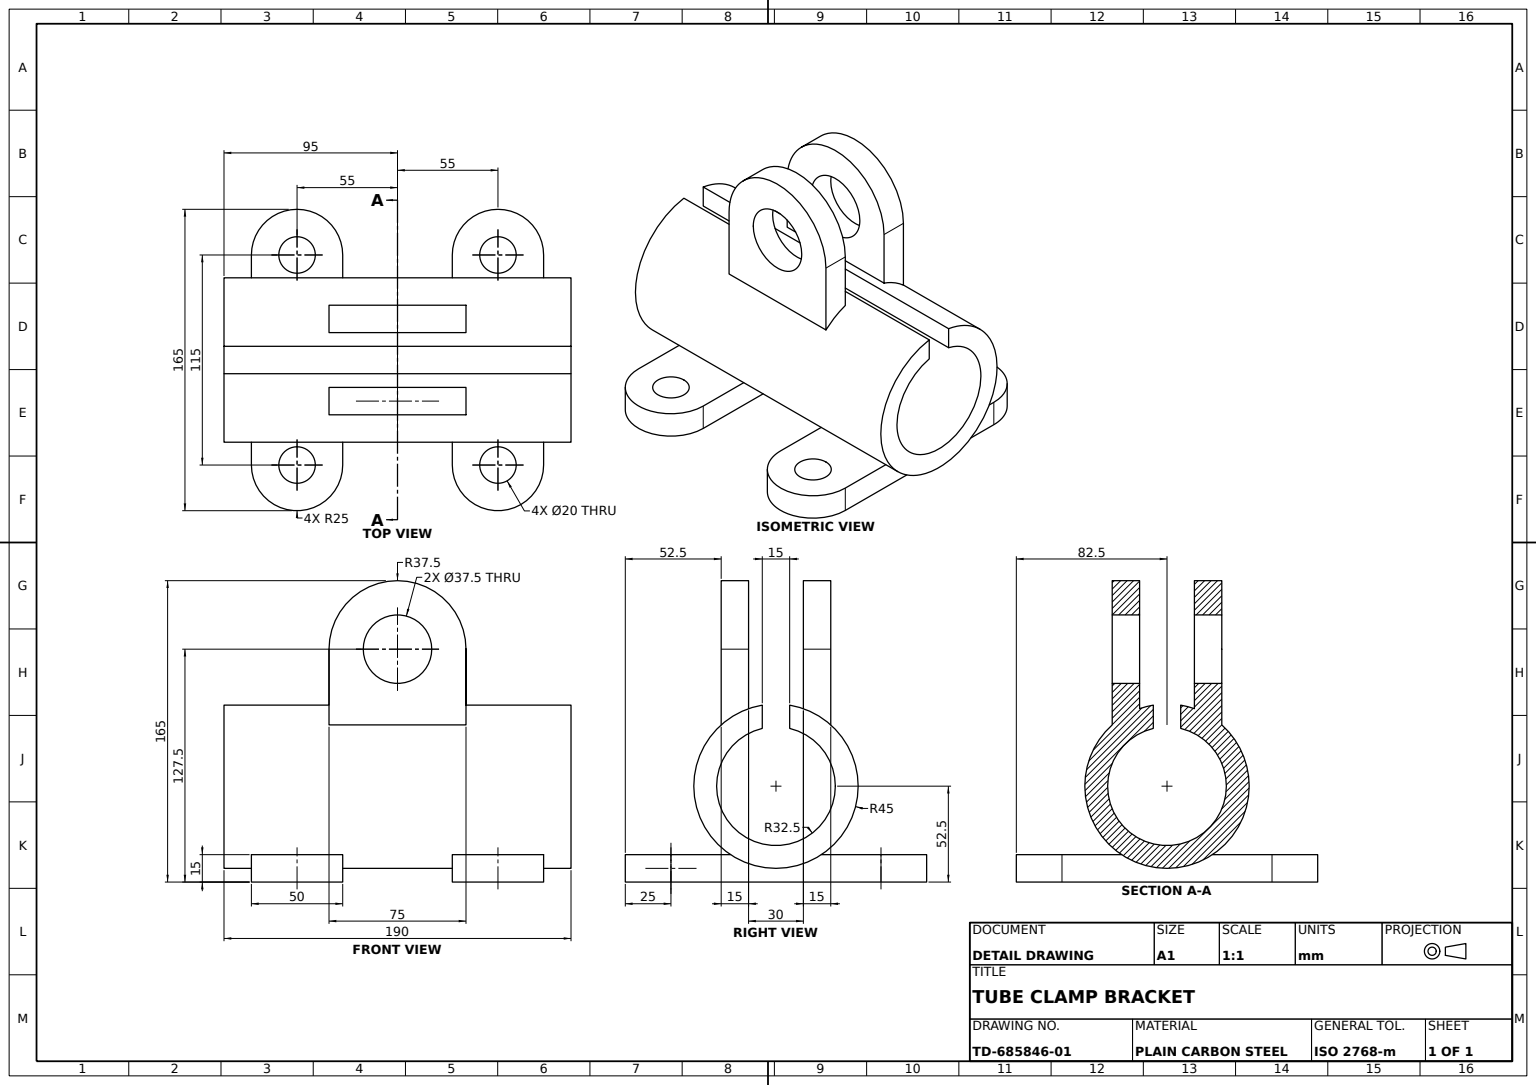
ISO-10303-21;
HEADER;
FILE_DESCRIPTION((''),'2;1');
FILE_NAME('','',(''),(''),'','','');
FILE_SCHEMA(('AUTOMOTIVE_DESIGN'));
ENDSEC;
DATA;
#1=APPLICATION_CONTEXT('');
#2=PRODUCT_CONTEXT('',#1,'mechanical');
#3=PRODUCT('','','',(#2));
#4=PRODUCT_DEFINITION_FORMATION('','',#3);
#5=PRODUCT_DEFINITION_CONTEXT('',#1,'design');
#6=PRODUCT_DEFINITION('','',#4,#5);
#7=PRODUCT_DEFINITION_SHAPE('','',#6);
#8=(LENGTH_UNIT()NAMED_UNIT(*)SI_UNIT(.MILLI.,.METRE.));
#9=(NAMED_UNIT(*)PLANE_ANGLE_UNIT()SI_UNIT($,.RADIAN.));
#10=(NAMED_UNIT(*)SI_UNIT($,.STERADIAN.)SOLID_ANGLE_UNIT());
#11=UNCERTAINTY_MEASURE_WITH_UNIT(LENGTH_MEASURE(1.E-05),#8,'distance_accuracy_value','');
#12=(GEOMETRIC_REPRESENTATION_CONTEXT(3)GLOBAL_UNCERTAINTY_ASSIGNED_CONTEXT((#11))GLOBAL_UNIT_ASSIGNED_CONTEXT((#8,#9,#10))REPRESENTATION_CONTEXT('',''));
#13=CARTESIAN_POINT('',(-55.,-37.5,67.5));
#14=VERTEX_POINT('',#13);
#15=CARTESIAN_POINT('',(-55.,-52.5,67.5));
#16=VERTEX_POINT('',#15);
#17=CARTESIAN_POINT('',(-55.,44.371598,67.5));
#18=DIRECTION('',(0.,-1.,0.));
#19=VECTOR('',#18,1000.);
#20=LINE('',#17,#19);
#21=EDGE_CURVE('',#14,#16,#20,.T.);
#22=ORIENTED_EDGE('',*,*,#21,.T.);
#23=CARTESIAN_POINT('',(-55.,-52.5,47.5));
#24=VERTEX_POINT('',#23);
#25=CARTESIAN_POINT('',(-55.,-52.5,57.5));
#26=DIRECTION('',(0.,0.,-1.));
#27=AXIS2_PLACEMENT_3D('',#25,#18,#26);
#28=CIRCLE('',#27,10.);
#29=EDGE_CURVE('',#16,#24,#28,.T.);
#30=ORIENTED_EDGE('',*,*,#29,.T.);
#31=CARTESIAN_POINT('',(-55.,-37.5,47.5));
#32=VERTEX_POINT('',#31);
#33=CARTESIAN_POINT('',(-55.,44.371598,47.5));
#34=LINE('',#33,#19);
#35=EDGE_CURVE('',#32,#24,#34,.T.);
#36=ORIENTED_EDGE('',*,*,#35,.F.);
#37=CARTESIAN_POINT('',(-55.,-37.5,57.5));
#38=DIRECTION('',(0.,1.,0.));
#39=AXIS2_PLACEMENT_3D('',#37,#38,#26);
#40=CIRCLE('',#39,10.);
#41=EDGE_CURVE('',#32,#14,#40,.T.);
#42=ORIENTED_EDGE('',*,*,#41,.T.);
#43=EDGE_LOOP('',(#22,#30,#36,#42));
#44=FACE_OUTER_BOUND('',#43,.T.);
#45=CARTESIAN_POINT('',(-55.,44.371598,57.5));
#46=AXIS2_PLACEMENT_3D('',#45,#18,#26);
#47=CYLINDRICAL_SURFACE('',#46,10.);
#48=ADVANCED_FACE('',(#44),#47,.F.);
#49=CARTESIAN_POINT('',(55.,-52.5,-82.5));
#50=VERTEX_POINT('',#49);
#51=CARTESIAN_POINT('',(80.,-52.5,-57.5));
#52=VERTEX_POINT('',#51);
#53=CARTESIAN_POINT('',(55.,-52.5,-57.5));
#54=AXIS2_PLACEMENT_3D('',#53,#18,#26);
#55=CIRCLE('',#54,25.);
#56=EDGE_CURVE('',#50,#52,#55,.T.);
#57=ORIENTED_EDGE('',*,*,#56,.T.);
#58=CARTESIAN_POINT('',(80.,-52.5,57.5));
#59=VERTEX_POINT('',#58);
#60=VECTOR('',#26,1000.);
#61=LINE('',#58,#60);
#62=EDGE_CURVE('',#59,#52,#61,.T.);
#63=ORIENTED_EDGE('',*,*,#62,.F.);
#64=CARTESIAN_POINT('',(30.,-52.5,57.5));
#65=VERTEX_POINT('',#64);
#66=CARTESIAN_POINT('',(55.,-52.5,57.5));
#67=DIRECTION('',(0.,0.,1.));
#68=AXIS2_PLACEMENT_3D('',#66,#38,#67);
#69=CIRCLE('',#68,25.);
#70=EDGE_CURVE('',#65,#59,#69,.T.);
#71=ORIENTED_EDGE('',*,*,#70,.F.);
#72=CARTESIAN_POINT('',(30.,-52.5,-57.5));
#73=VERTEX_POINT('',#72);
#74=LINE('',#64,#60);
#75=EDGE_CURVE('',#65,#73,#74,.T.);
#76=ORIENTED_EDGE('',*,*,#75,.T.);
#77=EDGE_CURVE('',#73,#50,#55,.T.);
#78=ORIENTED_EDGE('',*,*,#77,.T.);
#79=EDGE_LOOP('',(#57,#63,#71,#76,#78));
#80=FACE_OUTER_BOUND('',#79,.T.);
#81=CARTESIAN_POINT('',(55.,-52.5,-67.5));
#82=VERTEX_POINT('',#81);
#83=CARTESIAN_POINT('',(55.,-52.5,-47.5));
#84=VERTEX_POINT('',#83);
#85=CIRCLE('',#54,10.);
#86=EDGE_CURVE('',#82,#84,#85,.T.);
#87=ORIENTED_EDGE('',*,*,#86,.F.);
#88=EDGE_CURVE('',#84,#82,#85,.T.);
#89=ORIENTED_EDGE('',*,*,#88,.F.);
#90=EDGE_LOOP('',(#87,#89));
#91=FACE_BOUND('',#90,.T.);
#92=CARTESIAN_POINT('',(55.,-52.5,47.5));
#93=VERTEX_POINT('',#92);
#94=CARTESIAN_POINT('',(55.,-52.5,67.5));
#95=VERTEX_POINT('',#94);
#96=AXIS2_PLACEMENT_3D('',#66,#18,#26);
#97=CIRCLE('',#96,10.);
#98=EDGE_CURVE('',#93,#95,#97,.T.);
#99=ORIENTED_EDGE('',*,*,#98,.F.);
#100=EDGE_CURVE('',#95,#93,#97,.T.);
#101=ORIENTED_EDGE('',*,*,#100,.F.);
#102=EDGE_LOOP('',(#99,#101));
#103=FACE_BOUND('',#102,.T.);
#104=AXIS2_PLACEMENT_3D('',#58,#38,#67);
#105=PLANE('',#104);
#106=ADVANCED_FACE('',(#80,#91,#103),#105,.F.);
#107=CARTESIAN_POINT('',(-18.75,75.,-15.));
#108=VERTEX_POINT('',#107);
#109=CARTESIAN_POINT('',(18.75,75.,-15.));
#110=VERTEX_POINT('',#109);
#111=CARTESIAN_POINT('',(0.,75.,-15.));
#112=DIRECTION('',(1.,0.,0.));
#113=AXIS2_PLACEMENT_3D('',#111,#67,#112);
#114=CIRCLE('',#113,18.75);
#115=EDGE_CURVE('',#108,#110,#114,.T.);
#116=ORIENTED_EDGE('',*,*,#115,.F.);
#117=EDGE_CURVE('',#110,#108,#114,.T.);
#118=ORIENTED_EDGE('',*,*,#117,.F.);
#119=EDGE_LOOP('',(#116,#118));
#120=FACE_BOUND('',#119,.T.);
#121=CARTESIAN_POINT('',(37.5,75.,-15.));
#122=VERTEX_POINT('',#121);
#123=CARTESIAN_POINT('',(-37.5,75.,-15.));
#124=VERTEX_POINT('',#123);
#125=DIRECTION('',(-1.,0.,0.));
#126=AXIS2_PLACEMENT_3D('',#111,#67,#125);
#127=CIRCLE('',#126,37.5);
#128=EDGE_CURVE('',#122,#124,#127,.T.);
#129=ORIENTED_EDGE('',*,*,#128,.T.);
#130=CARTESIAN_POINT('',(-37.5,42.426407,-15.));
#131=VERTEX_POINT('',#130);
#132=LINE('',#123,#19);
#133=EDGE_CURVE('',#124,#131,#132,.T.);
#134=ORIENTED_EDGE('',*,*,#133,.T.);
#135=CARTESIAN_POINT('',(37.5,42.426407,-15.));
#136=VERTEX_POINT('',#135);
#137=CARTESIAN_POINT('',(95.,42.426407,-15.));
#138=VECTOR('',#125,1000.);
#139=LINE('',#137,#138);
#140=EDGE_CURVE('',#136,#131,#139,.T.);
#141=ORIENTED_EDGE('',*,*,#140,.F.);
#142=CARTESIAN_POINT('',(37.5,31.622777,-15.));
#143=VECTOR('',#38,1000.);
#144=LINE('',#142,#143);
#145=EDGE_CURVE('',#136,#122,#144,.T.);
#146=ORIENTED_EDGE('',*,*,#145,.T.);
#147=EDGE_LOOP('',(#129,#134,#141,#146));
#148=FACE_OUTER_BOUND('',#147,.T.);
#149=PLANE('',#126);
#150=ADVANCED_FACE('',(#120,#148),#149,.T.);
#151=CARTESIAN_POINT('',(80.,-37.5,-57.5));
#152=VERTEX_POINT('',#151);
#153=LINE('',#151,#143);
#154=EDGE_CURVE('',#52,#152,#153,.T.);
#155=ORIENTED_EDGE('',*,*,#154,.T.);
#156=CARTESIAN_POINT('',(80.,-37.5,-24.874686));
#157=VERTEX_POINT('',#156);
#158=CARTESIAN_POINT('',(80.,-37.5,57.5));
#159=LINE('',#158,#60);
#160=EDGE_CURVE('',#157,#152,#159,.T.);
#161=ORIENTED_EDGE('',*,*,#160,.F.);
#162=CARTESIAN_POINT('',(80.,-37.5,24.874686));
#163=VERTEX_POINT('',#162);
#164=CARTESIAN_POINT('',(80.,0.,0.));
#165=AXIS2_PLACEMENT_3D('',#164,#125,#67);
#166=CIRCLE('',#165,45.);
#167=EDGE_CURVE('',#157,#163,#166,.T.);
#168=ORIENTED_EDGE('',*,*,#167,.T.);
#169=VERTEX_POINT('',#158);
#170=EDGE_CURVE('',#169,#163,#159,.T.);
#171=ORIENTED_EDGE('',*,*,#170,.F.);
#172=LINE('',#158,#143);
#173=EDGE_CURVE('',#59,#169,#172,.T.);
#174=ORIENTED_EDGE('',*,*,#173,.F.);
#175=ORIENTED_EDGE('',*,*,#62,.T.);
#176=EDGE_LOOP('',(#155,#161,#168,#171,#174,#175));
#177=FACE_OUTER_BOUND('',#176,.T.);
#178=AXIS2_PLACEMENT_3D('',#158,#125,#67);
#179=PLANE('',#178);
#180=ADVANCED_FACE('',(#177),#179,.F.);
#181=CARTESIAN_POINT('',(-55.,-37.5,-67.5));
#182=VERTEX_POINT('',#181);
#183=CARTESIAN_POINT('',(-55.,-52.5,-67.5));
#184=VERTEX_POINT('',#183);
#185=CARTESIAN_POINT('',(-55.,44.371598,-67.5));
#186=LINE('',#185,#19);
#187=EDGE_CURVE('',#182,#184,#186,.T.);
#188=ORIENTED_EDGE('',*,*,#187,.F.);
#189=CARTESIAN_POINT('',(-55.,-37.5,-47.5));
#190=VERTEX_POINT('',#189);
#191=CARTESIAN_POINT('',(-55.,-37.5,-57.5));
#192=AXIS2_PLACEMENT_3D('',#191,#38,#26);
#193=CIRCLE('',#192,10.);
#194=EDGE_CURVE('',#182,#190,#193,.T.);
#195=ORIENTED_EDGE('',*,*,#194,.T.);
#196=CARTESIAN_POINT('',(-55.,-52.5,-47.5));
#197=VERTEX_POINT('',#196);
#198=CARTESIAN_POINT('',(-55.,44.371598,-47.5));
#199=LINE('',#198,#19);
#200=EDGE_CURVE('',#190,#197,#199,.T.);
#201=ORIENTED_EDGE('',*,*,#200,.T.);
#202=CARTESIAN_POINT('',(-55.,-52.5,-57.5));
#203=AXIS2_PLACEMENT_3D('',#202,#18,#26);
#204=CIRCLE('',#203,10.);
#205=EDGE_CURVE('',#197,#184,#204,.T.);
#206=ORIENTED_EDGE('',*,*,#205,.T.);
#207=EDGE_LOOP('',(#188,#195,#201,#206));
#208=FACE_OUTER_BOUND('',#207,.T.);
#209=CARTESIAN_POINT('',(-55.,44.371598,-57.5));
#210=AXIS2_PLACEMENT_3D('',#209,#18,#26);
#211=CYLINDRICAL_SURFACE('',#210,10.);
#212=ADVANCED_FACE('',(#208),#211,.F.);
#213=ORIENTED_EDGE('',*,*,#77,.F.);
#214=CARTESIAN_POINT('',(30.,-37.5,-57.5));
#215=VERTEX_POINT('',#214);
#216=LINE('',#214,#19);
#217=EDGE_CURVE('',#215,#73,#216,.T.);
#218=ORIENTED_EDGE('',*,*,#217,.F.);
#219=CARTESIAN_POINT('',(55.,-37.5,-82.5));
#220=VERTEX_POINT('',#219);
#221=CARTESIAN_POINT('',(55.,-37.5,-57.5));
#222=AXIS2_PLACEMENT_3D('',#221,#38,#26);
#223=CIRCLE('',#222,25.);
#224=EDGE_CURVE('',#220,#215,#223,.T.);
#225=ORIENTED_EDGE('',*,*,#224,.F.);
#226=CARTESIAN_POINT('',(55.,18.401699,-82.5));
#227=LINE('',#226,#19);
#228=EDGE_CURVE('',#220,#50,#227,.T.);
#229=ORIENTED_EDGE('',*,*,#228,.T.);
#230=EDGE_LOOP('',(#213,#218,#225,#229));
#231=FACE_OUTER_BOUND('',#230,.T.);
#232=CARTESIAN_POINT('',(55.,18.401699,-57.5));
#233=AXIS2_PLACEMENT_3D('',#232,#18,#26);
#234=CYLINDRICAL_SURFACE('',#233,25.);
#235=ADVANCED_FACE('',(#231),#234,.T.);
#236=ORIENTED_EDGE('',*,*,#98,.T.);
#237=CARTESIAN_POINT('',(55.,-37.5,67.5));
#238=VERTEX_POINT('',#237);
#239=CARTESIAN_POINT('',(55.,44.371598,67.5));
#240=LINE('',#239,#19);
#241=EDGE_CURVE('',#238,#95,#240,.T.);
#242=ORIENTED_EDGE('',*,*,#241,.F.);
#243=CARTESIAN_POINT('',(55.,-37.5,47.5));
#244=VERTEX_POINT('',#243);
#245=CARTESIAN_POINT('',(55.,-37.5,57.5));
#246=AXIS2_PLACEMENT_3D('',#245,#38,#26);
#247=CIRCLE('',#246,10.);
#248=EDGE_CURVE('',#238,#244,#247,.T.);
#249=ORIENTED_EDGE('',*,*,#248,.T.);
#250=CARTESIAN_POINT('',(55.,44.371598,47.5));
#251=LINE('',#250,#19);
#252=EDGE_CURVE('',#244,#93,#251,.T.);
#253=ORIENTED_EDGE('',*,*,#252,.T.);
#254=EDGE_LOOP('',(#236,#242,#249,#253));
#255=FACE_OUTER_BOUND('',#254,.T.);
#256=CARTESIAN_POINT('',(55.,44.371598,57.5));
#257=AXIS2_PLACEMENT_3D('',#256,#18,#26);
#258=CYLINDRICAL_SURFACE('',#257,10.);
#259=ADVANCED_FACE('',(#255),#258,.F.);
#260=ORIENTED_EDGE('',*,*,#115,.T.);
#261=CARTESIAN_POINT('',(18.75,75.,-30.));
#262=VERTEX_POINT('',#261);
#263=VECTOR('',#67,1000.);
#264=LINE('',#261,#263);
#265=EDGE_CURVE('',#262,#110,#264,.T.);
#266=ORIENTED_EDGE('',*,*,#265,.F.);
#267=CARTESIAN_POINT('',(-18.75,75.,-30.));
#268=VERTEX_POINT('',#267);
#269=CARTESIAN_POINT('',(0.,75.,-30.));
#270=AXIS2_PLACEMENT_3D('',#269,#67,#112);
#271=CIRCLE('',#270,18.75);
#272=EDGE_CURVE('',#268,#262,#271,.T.);
#273=ORIENTED_EDGE('',*,*,#272,.F.);
#274=LINE('',#267,#263);
#275=EDGE_CURVE('',#268,#108,#274,.T.);
#276=ORIENTED_EDGE('',*,*,#275,.T.);
#277=EDGE_LOOP('',(#260,#266,#273,#276));
#278=FACE_OUTER_BOUND('',#277,.T.);
#279=CYLINDRICAL_SURFACE('',#270,18.75);
#280=ADVANCED_FACE('',(#278),#279,.F.);
#281=CARTESIAN_POINT('',(30.,-37.5,24.874686));
#282=VERTEX_POINT('',#281);
#283=CARTESIAN_POINT('',(95.,-37.5,24.874686));
#284=LINE('',#283,#138);
#285=EDGE_CURVE('',#163,#282,#284,.T.);
#286=ORIENTED_EDGE('',*,*,#285,.T.);
#287=CARTESIAN_POINT('',(30.,-37.5,57.5));
#288=VERTEX_POINT('',#287);
#289=LINE('',#287,#60);
#290=EDGE_CURVE('',#288,#282,#289,.T.);
#291=ORIENTED_EDGE('',*,*,#290,.F.);
#292=AXIS2_PLACEMENT_3D('',#245,#18,#26);
#293=CIRCLE('',#292,25.);
#294=EDGE_CURVE('',#169,#288,#293,.T.);
#295=ORIENTED_EDGE('',*,*,#294,.F.);
#296=ORIENTED_EDGE('',*,*,#170,.T.);
#297=EDGE_LOOP('',(#286,#291,#295,#296));
#298=FACE_OUTER_BOUND('',#297,.T.);
#299=EDGE_CURVE('',#244,#238,#247,.T.);
#300=ORIENTED_EDGE('',*,*,#299,.F.);
#301=ORIENTED_EDGE('',*,*,#248,.F.);
#302=EDGE_LOOP('',(#300,#301));
#303=FACE_BOUND('',#302,.T.);
#304=AXIS2_PLACEMENT_3D('',#158,#18,#26);
#305=PLANE('',#304);
#306=ADVANCED_FACE('',(#298,#303),#305,.F.);
#307=CARTESIAN_POINT('',(95.,44.370598,-7.5));
#308=VERTEX_POINT('',#307);
#309=CARTESIAN_POINT('',(-95.,44.370598,-7.5));
#310=VERTEX_POINT('',#309);
#311=LINE('',#307,#138);
#312=EDGE_CURVE('',#308,#310,#311,.T.);
#313=ORIENTED_EDGE('',*,*,#312,.F.);
#314=CARTESIAN_POINT('',(95.,0.,-45.));
#315=VERTEX_POINT('',#314);
#316=CARTESIAN_POINT('',(95.,0.,0.));
#317=AXIS2_PLACEMENT_3D('',#316,#112,#67);
#318=CIRCLE('',#317,45.);
#319=EDGE_CURVE('',#315,#308,#318,.T.);
#320=ORIENTED_EDGE('',*,*,#319,.F.);
#321=CARTESIAN_POINT('',(-95.,0.,-45.));
#322=VERTEX_POINT('',#321);
#323=LINE('',#314,#138);
#324=EDGE_CURVE('',#315,#322,#323,.T.);
#325=ORIENTED_EDGE('',*,*,#324,.T.);
#326=CARTESIAN_POINT('',(-95.,0.,0.));
#327=AXIS2_PLACEMENT_3D('',#326,#112,#67);
#328=CIRCLE('',#327,45.);
#329=EDGE_CURVE('',#322,#310,#328,.T.);
#330=ORIENTED_EDGE('',*,*,#329,.T.);
#331=EDGE_LOOP('',(#313,#320,#325,#330));
#332=FACE_OUTER_BOUND('',#331,.T.);
#333=CARTESIAN_POINT('',(37.5,33.54102,-30.));
#334=VERTEX_POINT('',#333);
#335=CARTESIAN_POINT('',(37.5,0.,0.));
#336=AXIS2_PLACEMENT_3D('',#335,#112,#26);
#337=CIRCLE('',#336,45.);
#338=EDGE_CURVE('',#334,#136,#337,.T.);
#339=ORIENTED_EDGE('',*,*,#338,.T.);
#340=ORIENTED_EDGE('',*,*,#140,.T.);
#341=CARTESIAN_POINT('',(-37.5,33.54102,-30.));
#342=VERTEX_POINT('',#341);
#343=CARTESIAN_POINT('',(-37.5,0.,0.));
#344=AXIS2_PLACEMENT_3D('',#343,#125,#67);
#345=CIRCLE('',#344,45.);
#346=EDGE_CURVE('',#131,#342,#345,.T.);
#347=ORIENTED_EDGE('',*,*,#346,.T.);
#348=CARTESIAN_POINT('',(95.,33.54102,-30.));
#349=LINE('',#348,#138);
#350=EDGE_CURVE('',#334,#342,#349,.T.);
#351=ORIENTED_EDGE('',*,*,#350,.F.);
#352=EDGE_LOOP('',(#339,#340,#347,#351));
#353=FACE_BOUND('',#352,.T.);
#354=AXIS2_PLACEMENT_3D('',#316,#125,#67);
#355=CYLINDRICAL_SURFACE('',#354,45.);
#356=ADVANCED_FACE('',(#332,#353),#355,.T.);
#357=ORIENTED_EDGE('',*,*,#41,.F.);
#358=EDGE_CURVE('',#14,#32,#40,.T.);
#359=ORIENTED_EDGE('',*,*,#358,.F.);
#360=EDGE_LOOP('',(#357,#359));
#361=FACE_BOUND('',#360,.T.);
#362=CARTESIAN_POINT('',(-80.,-37.5,57.5));
#363=VERTEX_POINT('',#362);
#364=CARTESIAN_POINT('',(-80.,-37.5,24.874686));
#365=VERTEX_POINT('',#364);
#366=LINE('',#362,#60);
#367=EDGE_CURVE('',#363,#365,#366,.T.);
#368=ORIENTED_EDGE('',*,*,#367,.F.);
#369=CARTESIAN_POINT('',(-30.,-37.5,57.5));
#370=VERTEX_POINT('',#369);
#371=CIRCLE('',#39,25.);
#372=EDGE_CURVE('',#363,#370,#371,.T.);
#373=ORIENTED_EDGE('',*,*,#372,.T.);
#374=CARTESIAN_POINT('',(-30.,-37.5,24.874686));
#375=VERTEX_POINT('',#374);
#376=LINE('',#369,#60);
#377=EDGE_CURVE('',#370,#375,#376,.T.);
#378=ORIENTED_EDGE('',*,*,#377,.T.);
#379=EDGE_CURVE('',#375,#365,#284,.T.);
#380=ORIENTED_EDGE('',*,*,#379,.T.);
#381=EDGE_LOOP('',(#368,#373,#378,#380));
#382=FACE_OUTER_BOUND('',#381,.T.);
#383=AXIS2_PLACEMENT_3D('',#362,#18,#26);
#384=PLANE('',#383);
#385=ADVANCED_FACE('',(#361,#382),#384,.F.);
#386=CARTESIAN_POINT('',(95.,0.,-32.5));
#387=VERTEX_POINT('',#386);
#388=CARTESIAN_POINT('',(-95.,0.,-32.5));
#389=VERTEX_POINT('',#388);
#390=LINE('',#386,#138);
#391=EDGE_CURVE('',#387,#389,#390,.T.);
#392=ORIENTED_EDGE('',*,*,#391,.F.);
#393=CARTESIAN_POINT('',(95.,31.622777,-7.5));
#394=VERTEX_POINT('',#393);
#395=CIRCLE('',#354,32.5);
#396=EDGE_CURVE('',#394,#387,#395,.T.);
#397=ORIENTED_EDGE('',*,*,#396,.F.);
#398=CARTESIAN_POINT('',(-95.,31.622777,-7.5));
#399=VERTEX_POINT('',#398);
#400=LINE('',#393,#138);
#401=EDGE_CURVE('',#394,#399,#400,.T.);
#402=ORIENTED_EDGE('',*,*,#401,.T.);
#403=AXIS2_PLACEMENT_3D('',#326,#125,#67);
#404=CIRCLE('',#403,32.5);
#405=EDGE_CURVE('',#399,#389,#404,.T.);
#406=ORIENTED_EDGE('',*,*,#405,.T.);
#407=EDGE_LOOP('',(#392,#397,#402,#406));
#408=FACE_OUTER_BOUND('',#407,.T.);
#409=CYLINDRICAL_SURFACE('',#354,32.5);
#410=ADVANCED_FACE('',(#408),#409,.F.);
#411=CARTESIAN_POINT('',(-55.,-52.5,-82.5));
#412=VERTEX_POINT('',#411);
#413=CARTESIAN_POINT('',(-80.,-52.5,-57.5));
#414=VERTEX_POINT('',#413);
#415=AXIS2_PLACEMENT_3D('',#202,#38,#26);
#416=CIRCLE('',#415,25.);
#417=EDGE_CURVE('',#412,#414,#416,.T.);
#418=ORIENTED_EDGE('',*,*,#417,.T.);
#419=CARTESIAN_POINT('',(-80.,-37.5,-57.5));
#420=VERTEX_POINT('',#419);
#421=LINE('',#419,#19);
#422=EDGE_CURVE('',#420,#414,#421,.T.);
#423=ORIENTED_EDGE('',*,*,#422,.F.);
#424=CARTESIAN_POINT('',(-55.,-37.5,-82.5));
#425=VERTEX_POINT('',#424);
#426=AXIS2_PLACEMENT_3D('',#191,#18,#26);
#427=CIRCLE('',#426,25.);
#428=EDGE_CURVE('',#420,#425,#427,.T.);
#429=ORIENTED_EDGE('',*,*,#428,.T.);
#430=CARTESIAN_POINT('',(-55.,18.401699,-82.5));
#431=LINE('',#430,#19);
#432=EDGE_CURVE('',#425,#412,#431,.T.);
#433=ORIENTED_EDGE('',*,*,#432,.T.);
#434=EDGE_LOOP('',(#418,#423,#429,#433));
#435=FACE_OUTER_BOUND('',#434,.T.);
#436=CARTESIAN_POINT('',(-55.,18.401699,-57.5));
#437=AXIS2_PLACEMENT_3D('',#436,#18,#26);
#438=CYLINDRICAL_SURFACE('',#437,25.);
#439=ADVANCED_FACE('',(#435),#438,.T.);
#440=CARTESIAN_POINT('',(-37.5,75.,15.));
#441=VERTEX_POINT('',#440);
#442=CARTESIAN_POINT('',(-37.5,42.426407,15.));
#443=VERTEX_POINT('',#442);
#444=LINE('',#440,#19);
#445=EDGE_CURVE('',#441,#443,#444,.T.);
#446=ORIENTED_EDGE('',*,*,#445,.T.);
#447=CARTESIAN_POINT('',(-37.5,33.54102,30.));
#448=VERTEX_POINT('',#447);
#449=AXIS2_PLACEMENT_3D('',#343,#112,#26);
#450=CIRCLE('',#449,45.);
#451=EDGE_CURVE('',#443,#448,#450,.T.);
#452=ORIENTED_EDGE('',*,*,#451,.T.);
#453=CARTESIAN_POINT('',(-37.5,75.,30.));
#454=VERTEX_POINT('',#453);
#455=LINE('',#453,#19);
#456=EDGE_CURVE('',#454,#448,#455,.T.);
#457=ORIENTED_EDGE('',*,*,#456,.F.);
#458=LINE('',#453,#60);
#459=EDGE_CURVE('',#454,#441,#458,.T.);
#460=ORIENTED_EDGE('',*,*,#459,.T.);
#461=EDGE_LOOP('',(#446,#452,#457,#460));
#462=FACE_OUTER_BOUND('',#461,.T.);
#463=AXIS2_PLACEMENT_3D('',#453,#112,#26);
#464=PLANE('',#463);
#465=ADVANCED_FACE('',(#462),#464,.F.);
#466=CARTESIAN_POINT('',(-18.75,75.,30.));
#467=VERTEX_POINT('',#466);
#468=CARTESIAN_POINT('',(-18.75,75.,15.));
#469=VERTEX_POINT('',#468);
#470=LINE('',#466,#60);
#471=EDGE_CURVE('',#467,#469,#470,.T.);
#472=ORIENTED_EDGE('',*,*,#471,.T.);
#473=CARTESIAN_POINT('',(18.75,75.,15.));
#474=VERTEX_POINT('',#473);
#475=CARTESIAN_POINT('',(0.,75.,15.));
#476=AXIS2_PLACEMENT_3D('',#475,#67,#112);
#477=CIRCLE('',#476,18.75);
#478=EDGE_CURVE('',#474,#469,#477,.T.);
#479=ORIENTED_EDGE('',*,*,#478,.F.);
#480=CARTESIAN_POINT('',(18.75,75.,30.));
#481=VERTEX_POINT('',#480);
#482=LINE('',#480,#60);
#483=EDGE_CURVE('',#481,#474,#482,.T.);
#484=ORIENTED_EDGE('',*,*,#483,.F.);
#485=CARTESIAN_POINT('',(0.,75.,30.));
#486=AXIS2_PLACEMENT_3D('',#485,#67,#112);
#487=CIRCLE('',#486,18.75);
#488=EDGE_CURVE('',#481,#467,#487,.T.);
#489=ORIENTED_EDGE('',*,*,#488,.T.);
#490=EDGE_LOOP('',(#472,#479,#484,#489));
#491=FACE_OUTER_BOUND('',#490,.T.);
#492=AXIS2_PLACEMENT_3D('',#485,#26,#125);
#493=CYLINDRICAL_SURFACE('',#492,18.75);
#494=ADVANCED_FACE('',(#491),#493,.F.);
#495=CARTESIAN_POINT('',(-37.5,75.,-30.));
#496=VERTEX_POINT('',#495);
#497=LINE('',#495,#263);
#498=EDGE_CURVE('',#496,#124,#497,.T.);
#499=ORIENTED_EDGE('',*,*,#498,.F.);
#500=LINE('',#495,#19);
#501=EDGE_CURVE('',#496,#342,#500,.T.);
#502=ORIENTED_EDGE('',*,*,#501,.T.);
#503=ORIENTED_EDGE('',*,*,#346,.F.);
#504=ORIENTED_EDGE('',*,*,#133,.F.);
#505=EDGE_LOOP('',(#499,#502,#503,#504));
#506=FACE_OUTER_BOUND('',#505,.T.);
#507=AXIS2_PLACEMENT_3D('',#495,#125,#67);
#508=PLANE('',#507);
#509=ADVANCED_FACE('',(#506),#508,.T.);
#510=CARTESIAN_POINT('',(-30.,-37.5,-57.5));
#511=VERTEX_POINT('',#510);
#512=EDGE_CURVE('',#425,#511,#427,.T.);
#513=ORIENTED_EDGE('',*,*,#512,.T.);
#514=CARTESIAN_POINT('',(-30.,-52.5,-57.5));
#515=VERTEX_POINT('',#514);
#516=LINE('',#510,#143);
#517=EDGE_CURVE('',#515,#511,#516,.T.);
#518=ORIENTED_EDGE('',*,*,#517,.F.);
#519=EDGE_CURVE('',#515,#412,#416,.T.);
#520=ORIENTED_EDGE('',*,*,#519,.T.);
#521=ORIENTED_EDGE('',*,*,#432,.F.);
#522=EDGE_LOOP('',(#513,#518,#520,#521));
#523=FACE_OUTER_BOUND('',#522,.T.);
#524=ADVANCED_FACE('',(#523),#438,.T.);
#525=ORIENTED_EDGE('',*,*,#88,.T.);
#526=CARTESIAN_POINT('',(55.,-37.5,-67.5));
#527=VERTEX_POINT('',#526);
#528=CARTESIAN_POINT('',(55.,44.371598,-67.5));
#529=LINE('',#528,#19);
#530=EDGE_CURVE('',#527,#82,#529,.T.);
#531=ORIENTED_EDGE('',*,*,#530,.F.);
#532=CARTESIAN_POINT('',(55.,-37.5,-47.5));
#533=VERTEX_POINT('',#532);
#534=CIRCLE('',#222,10.);
#535=EDGE_CURVE('',#527,#533,#534,.T.);
#536=ORIENTED_EDGE('',*,*,#535,.T.);
#537=CARTESIAN_POINT('',(55.,44.371598,-47.5));
#538=LINE('',#537,#19);
#539=EDGE_CURVE('',#533,#84,#538,.T.);
#540=ORIENTED_EDGE('',*,*,#539,.T.);
#541=EDGE_LOOP('',(#525,#531,#536,#540));
#542=FACE_OUTER_BOUND('',#541,.T.);
#543=CARTESIAN_POINT('',(55.,44.371598,-57.5));
#544=AXIS2_PLACEMENT_3D('',#543,#18,#26);
#545=CYLINDRICAL_SURFACE('',#544,10.);
#546=ADVANCED_FACE('',(#542),#545,.F.);
#547=CARTESIAN_POINT('',(-80.,-52.5,57.5));
#548=VERTEX_POINT('',#547);
#549=LINE('',#362,#19);
#550=EDGE_CURVE('',#363,#548,#549,.T.);
#551=ORIENTED_EDGE('',*,*,#550,.F.);
#552=ORIENTED_EDGE('',*,*,#367,.T.);
#553=CARTESIAN_POINT('',(-80.,-37.5,-24.874686));
#554=VERTEX_POINT('',#553);
#555=CARTESIAN_POINT('',(-80.,0.,0.));
#556=AXIS2_PLACEMENT_3D('',#555,#112,#26);
#557=CIRCLE('',#556,45.);
#558=EDGE_CURVE('',#365,#554,#557,.T.);
#559=ORIENTED_EDGE('',*,*,#558,.T.);
#560=EDGE_CURVE('',#554,#420,#366,.T.);
#561=ORIENTED_EDGE('',*,*,#560,.T.);
#562=ORIENTED_EDGE('',*,*,#422,.T.);
#563=LINE('',#547,#60);
#564=EDGE_CURVE('',#548,#414,#563,.T.);
#565=ORIENTED_EDGE('',*,*,#564,.F.);
#566=EDGE_LOOP('',(#551,#552,#559,#561,#562,#565));
#567=FACE_OUTER_BOUND('',#566,.T.);
#568=AXIS2_PLACEMENT_3D('',#362,#112,#26);
#569=PLANE('',#568);
#570=ADVANCED_FACE('',(#567),#569,.F.);
#571=ORIENTED_EDGE('',*,*,#501,.F.);
#572=CARTESIAN_POINT('',(37.5,75.,-30.));
#573=VERTEX_POINT('',#572);
#574=AXIS2_PLACEMENT_3D('',#269,#67,#125);
#575=CIRCLE('',#574,37.5);
#576=EDGE_CURVE('',#573,#496,#575,.T.);
#577=ORIENTED_EDGE('',*,*,#576,.F.);
#578=CARTESIAN_POINT('',(37.5,31.622777,-30.));
#579=LINE('',#578,#143);
#580=EDGE_CURVE('',#334,#573,#579,.T.);
#581=ORIENTED_EDGE('',*,*,#580,.F.);
#582=ORIENTED_EDGE('',*,*,#350,.T.);
#583=EDGE_LOOP('',(#571,#577,#581,#582));
#584=FACE_OUTER_BOUND('',#583,.T.);
#585=ORIENTED_EDGE('',*,*,#272,.T.);
#586=EDGE_CURVE('',#262,#268,#271,.T.);
#587=ORIENTED_EDGE('',*,*,#586,.T.);
#588=EDGE_LOOP('',(#585,#587));
#589=FACE_BOUND('',#588,.T.);
#590=PLANE('',#574);
#591=ADVANCED_FACE('',(#584,#589),#590,.F.);
#592=EDGE_CURVE('',#184,#197,#204,.T.);
#593=ORIENTED_EDGE('',*,*,#592,.F.);
#594=ORIENTED_EDGE('',*,*,#205,.F.);
#595=EDGE_LOOP('',(#593,#594));
#596=FACE_BOUND('',#595,.T.);
#597=ORIENTED_EDGE('',*,*,#29,.F.);
#598=EDGE_CURVE('',#24,#16,#28,.T.);
#599=ORIENTED_EDGE('',*,*,#598,.F.);
#600=EDGE_LOOP('',(#597,#599));
#601=FACE_BOUND('',#600,.T.);
#602=ORIENTED_EDGE('',*,*,#417,.F.);
#603=ORIENTED_EDGE('',*,*,#519,.F.);
#604=CARTESIAN_POINT('',(-30.,-52.5,57.5));
#605=VERTEX_POINT('',#604);
#606=LINE('',#604,#60);
#607=EDGE_CURVE('',#605,#515,#606,.T.);
#608=ORIENTED_EDGE('',*,*,#607,.F.);
#609=AXIS2_PLACEMENT_3D('',#25,#18,#67);
#610=CIRCLE('',#609,25.);
#611=EDGE_CURVE('',#605,#548,#610,.T.);
#612=ORIENTED_EDGE('',*,*,#611,.T.);
#613=ORIENTED_EDGE('',*,*,#564,.T.);
#614=EDGE_LOOP('',(#602,#603,#608,#612,#613));
#615=FACE_OUTER_BOUND('',#614,.T.);
#616=AXIS2_PLACEMENT_3D('',#547,#38,#67);
#617=PLANE('',#616);
#618=ADVANCED_FACE('',(#596,#601,#615),#617,.F.);
#619=ORIENTED_EDGE('',*,*,#530,.T.);
#620=ORIENTED_EDGE('',*,*,#86,.T.);
#621=ORIENTED_EDGE('',*,*,#539,.F.);
#622=EDGE_CURVE('',#533,#527,#534,.T.);
#623=ORIENTED_EDGE('',*,*,#622,.T.);
#624=EDGE_LOOP('',(#619,#620,#621,#623));
#625=FACE_OUTER_BOUND('',#624,.T.);
#626=ADVANCED_FACE('',(#625),#545,.F.);
#627=ORIENTED_EDGE('',*,*,#228,.F.);
#628=EDGE_CURVE('',#152,#220,#223,.T.);
#629=ORIENTED_EDGE('',*,*,#628,.F.);
#630=ORIENTED_EDGE('',*,*,#154,.F.);
#631=ORIENTED_EDGE('',*,*,#56,.F.);
#632=EDGE_LOOP('',(#627,#629,#630,#631));
#633=FACE_OUTER_BOUND('',#632,.T.);
#634=ADVANCED_FACE('',(#633),#234,.T.);
#635=CARTESIAN_POINT('',(-95.,0.,32.5));
#636=VERTEX_POINT('',#635);
#637=EDGE_CURVE('',#389,#636,#404,.T.);
#638=ORIENTED_EDGE('',*,*,#637,.T.);
#639=CARTESIAN_POINT('',(95.,0.,32.5));
#640=VERTEX_POINT('',#639);
#641=LINE('',#639,#138);
#642=EDGE_CURVE('',#640,#636,#641,.T.);
#643=ORIENTED_EDGE('',*,*,#642,.F.);
#644=EDGE_CURVE('',#387,#640,#395,.T.);
#645=ORIENTED_EDGE('',*,*,#644,.F.);
#646=ORIENTED_EDGE('',*,*,#391,.T.);
#647=EDGE_LOOP('',(#638,#643,#645,#646));
#648=FACE_OUTER_BOUND('',#647,.T.);
#649=ADVANCED_FACE('',(#648),#409,.F.);
#650=CARTESIAN_POINT('',(37.5,33.54102,30.));
#651=VERTEX_POINT('',#650);
#652=CARTESIAN_POINT('',(95.,33.54102,30.));
#653=VECTOR('',#112,1000.);
#654=LINE('',#652,#653);
#655=EDGE_CURVE('',#448,#651,#654,.T.);
#656=ORIENTED_EDGE('',*,*,#655,.F.);
#657=ORIENTED_EDGE('',*,*,#451,.F.);
#658=CARTESIAN_POINT('',(37.5,42.426407,15.));
#659=VERTEX_POINT('',#658);
#660=CARTESIAN_POINT('',(95.,42.426407,15.));
#661=LINE('',#660,#653);
#662=EDGE_CURVE('',#443,#659,#661,.T.);
#663=ORIENTED_EDGE('',*,*,#662,.T.);
#664=AXIS2_PLACEMENT_3D('',#335,#125,#67);
#665=CIRCLE('',#664,45.);
#666=EDGE_CURVE('',#651,#659,#665,.T.);
#667=ORIENTED_EDGE('',*,*,#666,.F.);
#668=EDGE_LOOP('',(#656,#657,#663,#667));
#669=FACE_BOUND('',#668,.T.);
#670=CARTESIAN_POINT('',(-95.,44.370598,7.5));
#671=VERTEX_POINT('',#670);
#672=CARTESIAN_POINT('',(-95.,0.,45.));
#673=VERTEX_POINT('',#672);
#674=EDGE_CURVE('',#671,#673,#328,.T.);
#675=ORIENTED_EDGE('',*,*,#674,.T.);
#676=CARTESIAN_POINT('',(95.,0.,45.));
#677=VERTEX_POINT('',#676);
#678=LINE('',#676,#138);
#679=EDGE_CURVE('',#677,#673,#678,.T.);
#680=ORIENTED_EDGE('',*,*,#679,.F.);
#681=CARTESIAN_POINT('',(95.,44.370598,7.5));
#682=VERTEX_POINT('',#681);
#683=EDGE_CURVE('',#682,#677,#318,.T.);
#684=ORIENTED_EDGE('',*,*,#683,.F.);
#685=LINE('',#681,#138);
#686=EDGE_CURVE('',#682,#671,#685,.T.);
#687=ORIENTED_EDGE('',*,*,#686,.T.);
#688=EDGE_LOOP('',(#675,#680,#684,#687));
#689=FACE_OUTER_BOUND('',#688,.T.);
#690=ADVANCED_FACE('',(#669,#689),#355,.T.);
#691=ORIENTED_EDGE('',*,*,#642,.T.);
#692=CARTESIAN_POINT('',(-95.,31.622777,7.5));
#693=VERTEX_POINT('',#692);
#694=EDGE_CURVE('',#636,#693,#404,.T.);
#695=ORIENTED_EDGE('',*,*,#694,.T.);
#696=CARTESIAN_POINT('',(95.,31.622777,7.5));
#697=VERTEX_POINT('',#696);
#698=LINE('',#696,#138);
#699=EDGE_CURVE('',#697,#693,#698,.T.);
#700=ORIENTED_EDGE('',*,*,#699,.F.);
#701=EDGE_CURVE('',#640,#697,#395,.T.);
#702=ORIENTED_EDGE('',*,*,#701,.F.);
#703=EDGE_LOOP('',(#691,#695,#700,#702));
#704=FACE_OUTER_BOUND('',#703,.T.);
#705=ADVANCED_FACE('',(#704),#409,.F.);
#706=ORIENTED_EDGE('',*,*,#377,.F.);
#707=LINE('',#369,#143);
#708=EDGE_CURVE('',#605,#370,#707,.T.);
#709=ORIENTED_EDGE('',*,*,#708,.F.);
#710=ORIENTED_EDGE('',*,*,#607,.T.);
#711=ORIENTED_EDGE('',*,*,#517,.T.);
#712=CARTESIAN_POINT('',(-30.,-37.5,-24.874686));
#713=VERTEX_POINT('',#712);
#714=EDGE_CURVE('',#713,#511,#376,.T.);
#715=ORIENTED_EDGE('',*,*,#714,.F.);
#716=CARTESIAN_POINT('',(-30.,0.,0.));
#717=AXIS2_PLACEMENT_3D('',#716,#125,#67);
#718=CIRCLE('',#717,45.);
#719=EDGE_CURVE('',#713,#375,#718,.T.);
#720=ORIENTED_EDGE('',*,*,#719,.T.);
#721=EDGE_LOOP('',(#706,#709,#710,#711,#715,#720));
#722=FACE_OUTER_BOUND('',#721,.T.);
#723=AXIS2_PLACEMENT_3D('',#369,#125,#67);
#724=PLANE('',#723);
#725=ADVANCED_FACE('',(#722),#724,.F.);
#726=CARTESIAN_POINT('',(37.5,75.,30.));
#727=VERTEX_POINT('',#726);
#728=CARTESIAN_POINT('',(37.5,75.,15.));
#729=VERTEX_POINT('',#728);
#730=LINE('',#726,#60);
#731=EDGE_CURVE('',#727,#729,#730,.T.);
#732=ORIENTED_EDGE('',*,*,#731,.T.);
#733=AXIS2_PLACEMENT_3D('',#475,#67,#125);
#734=CIRCLE('',#733,37.5);
#735=EDGE_CURVE('',#729,#441,#734,.T.);
#736=ORIENTED_EDGE('',*,*,#735,.T.);
#737=ORIENTED_EDGE('',*,*,#459,.F.);
#738=AXIS2_PLACEMENT_3D('',#485,#67,#125);
#739=CIRCLE('',#738,37.5);
#740=EDGE_CURVE('',#727,#454,#739,.T.);
#741=ORIENTED_EDGE('',*,*,#740,.F.);
#742=EDGE_LOOP('',(#732,#736,#737,#741));
#743=FACE_OUTER_BOUND('',#742,.T.);
#744=CYLINDRICAL_SURFACE('',#492,37.5);
#745=ADVANCED_FACE('',(#743),#744,.T.);
#746=ORIENTED_EDGE('',*,*,#290,.T.);
#747=CARTESIAN_POINT('',(30.,-37.5,-24.874686));
#748=VERTEX_POINT('',#747);
#749=CARTESIAN_POINT('',(30.,0.,0.));
#750=AXIS2_PLACEMENT_3D('',#749,#112,#26);
#751=CIRCLE('',#750,45.);
#752=EDGE_CURVE('',#282,#748,#751,.T.);
#753=ORIENTED_EDGE('',*,*,#752,.T.);
#754=EDGE_CURVE('',#748,#215,#289,.T.);
#755=ORIENTED_EDGE('',*,*,#754,.T.);
#756=ORIENTED_EDGE('',*,*,#217,.T.);
#757=ORIENTED_EDGE('',*,*,#75,.F.);
#758=LINE('',#287,#19);
#759=EDGE_CURVE('',#288,#65,#758,.T.);
#760=ORIENTED_EDGE('',*,*,#759,.F.);
#761=EDGE_LOOP('',(#746,#753,#755,#756,#757,#760));
#762=FACE_OUTER_BOUND('',#761,.T.);
#763=AXIS2_PLACEMENT_3D('',#287,#112,#26);
#764=PLANE('',#763);
#765=ADVANCED_FACE('',(#762),#764,.F.);
#766=ORIENTED_EDGE('',*,*,#754,.F.);
#767=CARTESIAN_POINT('',(95.,-37.5,-24.874686));
#768=LINE('',#767,#653);
#769=EDGE_CURVE('',#748,#157,#768,.T.);
#770=ORIENTED_EDGE('',*,*,#769,.T.);
#771=ORIENTED_EDGE('',*,*,#160,.T.);
#772=ORIENTED_EDGE('',*,*,#628,.T.);
#773=ORIENTED_EDGE('',*,*,#224,.T.);
#774=EDGE_LOOP('',(#766,#770,#771,#772,#773));
#775=FACE_OUTER_BOUND('',#774,.T.);
#776=ORIENTED_EDGE('',*,*,#535,.F.);
#777=ORIENTED_EDGE('',*,*,#622,.F.);
#778=EDGE_LOOP('',(#776,#777));
#779=FACE_BOUND('',#778,.T.);
#780=ADVANCED_FACE('',(#775,#779),#305,.F.);
#781=ORIENTED_EDGE('',*,*,#731,.F.);
#782=CARTESIAN_POINT('',(37.5,31.622777,30.));
#783=LINE('',#782,#143);
#784=EDGE_CURVE('',#651,#727,#783,.T.);
#785=ORIENTED_EDGE('',*,*,#784,.F.);
#786=ORIENTED_EDGE('',*,*,#666,.T.);
#787=CARTESIAN_POINT('',(37.5,31.622777,15.));
#788=LINE('',#787,#143);
#789=EDGE_CURVE('',#659,#729,#788,.T.);
#790=ORIENTED_EDGE('',*,*,#789,.T.);
#791=EDGE_LOOP('',(#781,#785,#786,#790));
#792=FACE_OUTER_BOUND('',#791,.T.);
#793=AXIS2_PLACEMENT_3D('',#782,#125,#67);
#794=PLANE('',#793);
#795=ADVANCED_FACE('',(#792),#794,.F.);
#796=ORIENTED_EDGE('',*,*,#187,.T.);
#797=ORIENTED_EDGE('',*,*,#592,.T.);
#798=ORIENTED_EDGE('',*,*,#200,.F.);
#799=EDGE_CURVE('',#190,#182,#193,.T.);
#800=ORIENTED_EDGE('',*,*,#799,.T.);
#801=EDGE_LOOP('',(#796,#797,#798,#800));
#802=FACE_OUTER_BOUND('',#801,.T.);
#803=ADVANCED_FACE('',(#802),#211,.F.);
#804=ORIENTED_EDGE('',*,*,#35,.T.);
#805=ORIENTED_EDGE('',*,*,#598,.T.);
#806=ORIENTED_EDGE('',*,*,#21,.F.);
#807=ORIENTED_EDGE('',*,*,#358,.T.);
#808=EDGE_LOOP('',(#804,#805,#806,#807));
#809=FACE_OUTER_BOUND('',#808,.T.);
#810=ADVANCED_FACE('',(#809),#47,.F.);
#811=ORIENTED_EDGE('',*,*,#662,.F.);
#812=ORIENTED_EDGE('',*,*,#445,.F.);
#813=ORIENTED_EDGE('',*,*,#735,.F.);
#814=ORIENTED_EDGE('',*,*,#789,.F.);
#815=EDGE_LOOP('',(#811,#812,#813,#814));
#816=FACE_OUTER_BOUND('',#815,.T.);
#817=EDGE_CURVE('',#469,#474,#477,.T.);
#818=ORIENTED_EDGE('',*,*,#817,.T.);
#819=ORIENTED_EDGE('',*,*,#478,.T.);
#820=EDGE_LOOP('',(#818,#819));
#821=FACE_BOUND('',#820,.T.);
#822=AXIS2_PLACEMENT_3D('',#475,#26,#125);
#823=PLANE('',#822);
#824=ADVANCED_FACE('',(#816,#821),#823,.T.);
#825=LINE('',#307,#19);
#826=EDGE_CURVE('',#308,#394,#825,.T.);
#827=ORIENTED_EDGE('',*,*,#826,.F.);
#828=ORIENTED_EDGE('',*,*,#312,.T.);
#829=LINE('',#309,#19);
#830=EDGE_CURVE('',#310,#399,#829,.T.);
#831=ORIENTED_EDGE('',*,*,#830,.T.);
#832=ORIENTED_EDGE('',*,*,#401,.F.);
#833=EDGE_LOOP('',(#827,#828,#831,#832));
#834=FACE_OUTER_BOUND('',#833,.T.);
#835=AXIS2_PLACEMENT_3D('',#307,#26,#125);
#836=PLANE('',#835);
#837=ADVANCED_FACE('',(#834),#836,.F.);
#838=ORIENTED_EDGE('',*,*,#471,.F.);
#839=EDGE_CURVE('',#467,#481,#487,.T.);
#840=ORIENTED_EDGE('',*,*,#839,.T.);
#841=ORIENTED_EDGE('',*,*,#483,.T.);
#842=ORIENTED_EDGE('',*,*,#817,.F.);
#843=EDGE_LOOP('',(#838,#840,#841,#842));
#844=FACE_OUTER_BOUND('',#843,.T.);
#845=ADVANCED_FACE('',(#844),#493,.F.);
#846=ORIENTED_EDGE('',*,*,#117,.T.);
#847=ORIENTED_EDGE('',*,*,#275,.F.);
#848=ORIENTED_EDGE('',*,*,#586,.F.);
#849=ORIENTED_EDGE('',*,*,#265,.T.);
#850=EDGE_LOOP('',(#846,#847,#848,#849));
#851=FACE_OUTER_BOUND('',#850,.T.);
#852=ADVANCED_FACE('',(#851),#279,.F.);
#853=ORIENTED_EDGE('',*,*,#379,.F.);
#854=ORIENTED_EDGE('',*,*,#719,.F.);
#855=EDGE_CURVE('',#554,#713,#768,.T.);
#856=ORIENTED_EDGE('',*,*,#855,.F.);
#857=ORIENTED_EDGE('',*,*,#558,.F.);
#858=EDGE_LOOP('',(#853,#854,#856,#857));
#859=FACE_BOUND('',#858,.T.);
#860=ORIENTED_EDGE('',*,*,#285,.F.);
#861=ORIENTED_EDGE('',*,*,#167,.F.);
#862=ORIENTED_EDGE('',*,*,#769,.F.);
#863=ORIENTED_EDGE('',*,*,#752,.F.);
#864=EDGE_LOOP('',(#860,#861,#862,#863));
#865=FACE_BOUND('',#864,.T.);
#866=EDGE_CURVE('',#673,#322,#328,.T.);
#867=ORIENTED_EDGE('',*,*,#866,.T.);
#868=ORIENTED_EDGE('',*,*,#324,.F.);
#869=EDGE_CURVE('',#677,#315,#318,.T.);
#870=ORIENTED_EDGE('',*,*,#869,.F.);
#871=ORIENTED_EDGE('',*,*,#679,.T.);
#872=EDGE_LOOP('',(#867,#868,#870,#871));
#873=FACE_OUTER_BOUND('',#872,.T.);
#874=ADVANCED_FACE('',(#859,#865,#873),#355,.T.);
#875=ORIENTED_EDGE('',*,*,#759,.T.);
#876=ORIENTED_EDGE('',*,*,#70,.T.);
#877=ORIENTED_EDGE('',*,*,#173,.T.);
#878=ORIENTED_EDGE('',*,*,#294,.T.);
#879=EDGE_LOOP('',(#875,#876,#877,#878));
#880=FACE_OUTER_BOUND('',#879,.T.);
#881=CARTESIAN_POINT('',(55.,18.401699,57.5));
#882=AXIS2_PLACEMENT_3D('',#881,#18,#26);
#883=CYLINDRICAL_SURFACE('',#882,25.);
#884=ADVANCED_FACE('',(#880),#883,.T.);
#885=ORIENTED_EDGE('',*,*,#319,.T.);
#886=ORIENTED_EDGE('',*,*,#826,.T.);
#887=ORIENTED_EDGE('',*,*,#396,.T.);
#888=ORIENTED_EDGE('',*,*,#644,.T.);
#889=ORIENTED_EDGE('',*,*,#701,.T.);
#890=LINE('',#681,#143);
#891=EDGE_CURVE('',#697,#682,#890,.T.);
#892=ORIENTED_EDGE('',*,*,#891,.T.);
#893=ORIENTED_EDGE('',*,*,#683,.T.);
#894=ORIENTED_EDGE('',*,*,#869,.T.);
#895=EDGE_LOOP('',(#885,#886,#887,#888,#889,#892,#893,#894));
#896=FACE_OUTER_BOUND('',#895,.T.);
#897=PLANE('',#354);
#898=ADVANCED_FACE('',(#896),#897,.F.);
#899=ORIENTED_EDGE('',*,*,#694,.F.);
#900=ORIENTED_EDGE('',*,*,#637,.F.);
#901=ORIENTED_EDGE('',*,*,#405,.F.);
#902=ORIENTED_EDGE('',*,*,#830,.F.);
#903=ORIENTED_EDGE('',*,*,#329,.F.);
#904=ORIENTED_EDGE('',*,*,#866,.F.);
#905=ORIENTED_EDGE('',*,*,#674,.F.);
#906=LINE('',#670,#143);
#907=EDGE_CURVE('',#693,#671,#906,.T.);
#908=ORIENTED_EDGE('',*,*,#907,.F.);
#909=EDGE_LOOP('',(#899,#900,#901,#902,#903,#904,#905,#908));
#910=FACE_OUTER_BOUND('',#909,.T.);
#911=PLANE('',#403);
#912=ADVANCED_FACE('',(#910),#911,.T.);
#913=LINE('',#572,#263);
#914=EDGE_CURVE('',#573,#122,#913,.T.);
#915=ORIENTED_EDGE('',*,*,#914,.F.);
#916=ORIENTED_EDGE('',*,*,#576,.T.);
#917=ORIENTED_EDGE('',*,*,#498,.T.);
#918=ORIENTED_EDGE('',*,*,#128,.F.);
#919=EDGE_LOOP('',(#915,#916,#917,#918));
#920=FACE_OUTER_BOUND('',#919,.T.);
#921=CYLINDRICAL_SURFACE('',#270,37.5);
#922=ADVANCED_FACE('',(#920),#921,.T.);
#923=ORIENTED_EDGE('',*,*,#799,.F.);
#924=ORIENTED_EDGE('',*,*,#194,.F.);
#925=EDGE_LOOP('',(#923,#924));
#926=FACE_BOUND('',#925,.T.);
#927=ORIENTED_EDGE('',*,*,#512,.F.);
#928=ORIENTED_EDGE('',*,*,#428,.F.);
#929=ORIENTED_EDGE('',*,*,#560,.F.);
#930=ORIENTED_EDGE('',*,*,#855,.T.);
#931=ORIENTED_EDGE('',*,*,#714,.T.);
#932=EDGE_LOOP('',(#927,#928,#929,#930,#931));
#933=FACE_OUTER_BOUND('',#932,.T.);
#934=ADVANCED_FACE('',(#926,#933),#384,.F.);
#935=ORIENTED_EDGE('',*,*,#914,.T.);
#936=ORIENTED_EDGE('',*,*,#145,.F.);
#937=ORIENTED_EDGE('',*,*,#338,.F.);
#938=ORIENTED_EDGE('',*,*,#580,.T.);
#939=EDGE_LOOP('',(#935,#936,#937,#938));
#940=FACE_OUTER_BOUND('',#939,.T.);
#941=AXIS2_PLACEMENT_3D('',#578,#112,#26);
#942=PLANE('',#941);
#943=ADVANCED_FACE('',(#940),#942,.T.);
#944=ORIENTED_EDGE('',*,*,#252,.F.);
#945=ORIENTED_EDGE('',*,*,#299,.T.);
#946=ORIENTED_EDGE('',*,*,#241,.T.);
#947=ORIENTED_EDGE('',*,*,#100,.T.);
#948=EDGE_LOOP('',(#944,#945,#946,#947));
#949=FACE_OUTER_BOUND('',#948,.T.);
#950=ADVANCED_FACE('',(#949),#258,.F.);
#951=ORIENTED_EDGE('',*,*,#372,.F.);
#952=ORIENTED_EDGE('',*,*,#550,.T.);
#953=ORIENTED_EDGE('',*,*,#611,.F.);
#954=ORIENTED_EDGE('',*,*,#708,.T.);
#955=EDGE_LOOP('',(#951,#952,#953,#954));
#956=FACE_OUTER_BOUND('',#955,.T.);
#957=CARTESIAN_POINT('',(-55.,18.401699,57.5));
#958=AXIS2_PLACEMENT_3D('',#957,#18,#26);
#959=CYLINDRICAL_SURFACE('',#958,25.);
#960=ADVANCED_FACE('',(#956),#959,.T.);
#961=ORIENTED_EDGE('',*,*,#891,.F.);
#962=ORIENTED_EDGE('',*,*,#699,.T.);
#963=ORIENTED_EDGE('',*,*,#907,.T.);
#964=ORIENTED_EDGE('',*,*,#686,.F.);
#965=EDGE_LOOP('',(#961,#962,#963,#964));
#966=FACE_OUTER_BOUND('',#965,.T.);
#967=AXIS2_PLACEMENT_3D('',#681,#67,#112);
#968=PLANE('',#967);
#969=ADVANCED_FACE('',(#966),#968,.F.);
#970=ORIENTED_EDGE('',*,*,#784,.T.);
#971=ORIENTED_EDGE('',*,*,#740,.T.);
#972=ORIENTED_EDGE('',*,*,#456,.T.);
#973=ORIENTED_EDGE('',*,*,#655,.T.);
#974=EDGE_LOOP('',(#970,#971,#972,#973));
#975=FACE_OUTER_BOUND('',#974,.T.);
#976=ORIENTED_EDGE('',*,*,#488,.F.);
#977=ORIENTED_EDGE('',*,*,#839,.F.);
#978=EDGE_LOOP('',(#976,#977));
#979=FACE_BOUND('',#978,.T.);
#980=PLANE('',#492);
#981=ADVANCED_FACE('',(#975,#979),#980,.F.);
#982=CLOSED_SHELL('',(#48,#106,#150,#180,#212,#235,#259,#280,#306,#356,#385,#410,#439,#465,#494,#509,#524,#546,#570,#591,#618,#626,#634,#649,#690,#705,#725,#745,#765,#780,#795,#803,#810,#824,#837,#845,#852,#874,#884,#898,#912,#922,#934,#943,#950,#960,#969,#981));
#983=MANIFOLD_SOLID_BREP('',#982);
#984=ADVANCED_BREP_SHAPE_REPRESENTATION('',(#983),#12);
#985=SHAPE_DEFINITION_REPRESENTATION(#7,#984);
ENDSEC;
END-ISO-10303-21;
